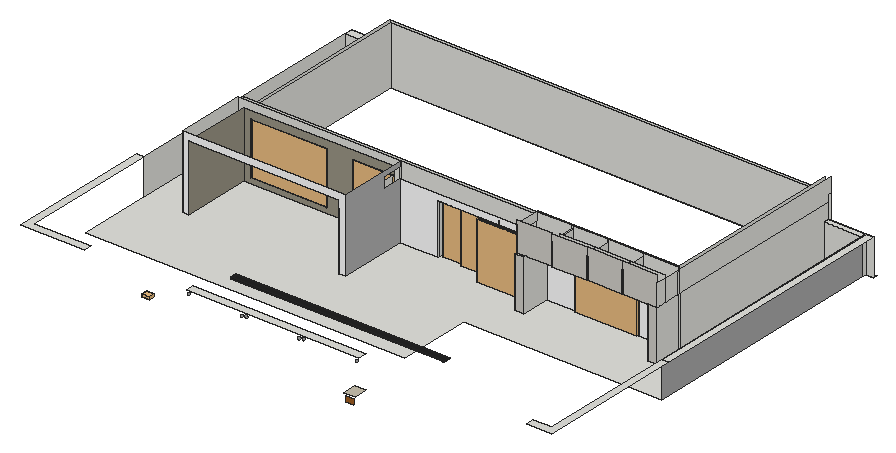
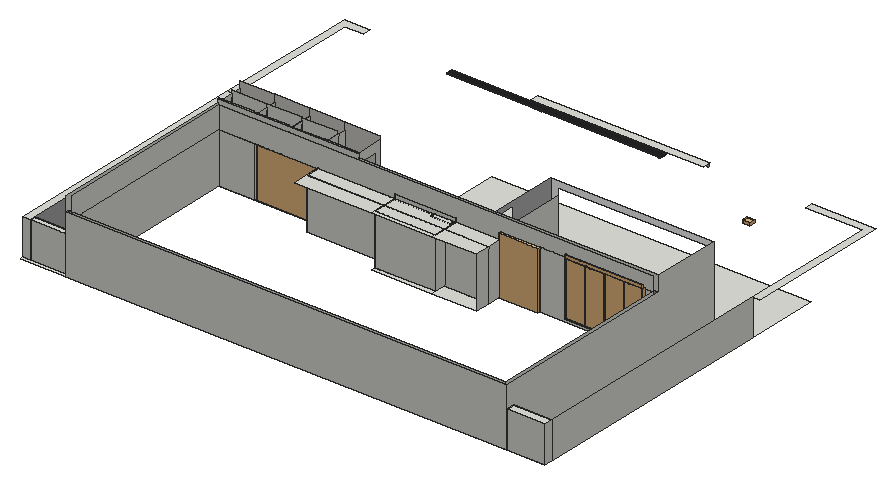
# SketchUp Ruby script. Lengths in inches.
U = 1.inch
M = Sketchup.active_model
def pt(a) = Geom::Point3d.new(a.map { |v| v * U })
def face(e, loops, mat)
  f = e.add_face(loops[0].map { |a| pt(a) })
  loops[1..].each { |l| e.add_face(l.map { |a| pt(a) }).erase! }
  f.material = f.back_material = mat if mat
  f
end
# faces: each face lists its corners as indices into pts; further lists are holes
def faces(e, pts, list, mat = nil) = list.each { |f| face(e, (f[0].is_a?(Array) ? f : [f]).map { |l| l.map { |i| pts[i] } }, mat) }
# xy, xz, yz: faces in a plane at the given z, y or x. An outline is a flat list of corners, or four numbers for a rectangle; further outlines are holes
def ring(l) = l.size == 4 ? [[l[0], l[1]], [l[2], l[1]], [l[2], l[3]], [l[0], l[3]]] : l.each_slice(2).to_a
def flat(e, list, mat, &to3) = list.each { |f| face(e, (f[0].is_a?(Array) ? f : [f]).map { |l| ring(l).map { |u, v| to3.(u, v) } }, mat) }
def xy(e, z, list, mat = nil) = flat(e, list, mat) { |x, y| [x, y, z] }
def xz(e, y, list, mat = nil) = flat(e, list, mat) { |x, z| [x, y, z] }
def yz(e, x, list, mat = nil) = flat(e, list, mat) { |y, z| [x, y, z] }
def lines(e, pts, list) = list.each { |a, b| e.add_line(pt(pts[a]), pt(pts[b])) }
# prism: a flat outline (further loops are holes) pulled along v
def prism(e, loops, v, mat = nil)
  f = face(e, loops, mat); d = Geom::Vector3d.new(v.map { |x| x * U })
  f.pushpull(f.normal.samedirection?(d) ? d.length : -d.length)
end
def box(e, o, s, mat = nil) = prism(e, [[o, [o[0] + s[0], o[1], o[2]], [o[0] + s[0], o[1] + s[1], o[2]], [o[0], o[1] + s[1], o[2]]]], [0, 0, s[2]], mat)
def at(x, y, z, deg = 0) = Geom::Transformation.translation(pt([x, y, z])) * Geom::Transformation.rotation(ORIGIN, Z_AXIS, deg.degrees)
def axes(o, x, y, z) = Geom::Transformation.new([*x, 0, *y, 0, *z, 0, *pt(o).to_a, 1])
def part(name) = M.definitions.add(name)
# library, detail: a bought-in or finely detailed component or shape, given as its bounding box
def library(name, o, s) = part(name).tap { |d| box(d.entities, o, s) }
def detail(e, o, s) = box(e.add_group.entities, o, s)
def put(e, d, t, mat = nil) = e.add_instance(d, t).tap { |i| i.material = mat if mat }
def group(e, t, mat = nil) = e.add_group.tap { |g| g.transformation = t; g.material = mat if mat }.entities
root = M.entities
M.materials.add("Material~3").color = [123, 113, 102]
M.materials.add("[0128_White]").color = [255, 255, 255]
M.materials.add("[0129_WhiteSmoke]").color = [178, 178, 178]
M.materials.add("[0132_LightGray]").color = [169, 169, 169]
M.materials.add("[0136_Charcoal]").color = [35, 35, 35]
M.materials.add("[Concrete Tile]").color = [155, 150, 134]
M.materials.add("[Terrazzo Tile Light]").color = [209, 207, 200]
M.materials.add("[Tile Canvas]").color = [199, 192, 173]
M.materials.add("[Wood Square Tile 02]").color = [160, 95, 34]
M.materials.add("terracota").color = [125, 74, 68]
c1 = library("3DGeom~4_Defintion",[362.52,-15.59,12.6],[288.85,70.11,1000])
c2 = library("3 door",[0,0,0],[74.8,3.9375,43.31])
c3 = library("Shallow planter bowl",[0,0,0],[21.33,16.65,7.48])
c4 = library("door (1)",[38.93,25.48,0],[40,9.94,82.68])
c5 = part("Group\#105")
prism(c5.entities,[[[353.71,0,0.79],[353.71,0,-1.18],[353.71,10.43,-1.18],[353.71,10.43,0.79],[353.71,10.12,0.79],[353.71,10.12,0.39],[353.71,7.09,0.39],[353.71,7.09,0.79],[353.71,6.73,0.79],[353.71,6.73,0.39],[353.71,3.7,0.39],[353.71,3.7,0.79],[353.71,3.35,0.79],[353.71,3.35,0.39],[353.71,0.31,0.39],[353.71,0.31,0.79]]],[-353.71,0,0])
c6 = library("JALI+PATTERN-03",[8.875,53.125,6.4375],[84,1,53.5])
xy(root,5.1875,[[[1168.49,611.53,1696.41,611.53,1696.41,732.28,2024.12,732.28,2024.12,1146.63,1960.87,1146.63,1960.87,851.0625,1791.45,851.0625,1791.45,845.35,1744,845.35,1744,798.41,1728.67,798.41,1728.67,845.35,1664.38,845.35,1664.38,874.25,1564.1,874.25,1564.1,845.35,1501.42,845.35,1501.42,732.28,1490.48,732.28,1490.48,851.0625,1425.1,851.0625,1425.1,845.35,1243.06,845.35,1243.06,732.28,1232.12,732.28,1232.12,1146.63,1168.49,1146.63],[1945.54,801.78,1960.87,845.35]],[1232.12,732.28,1232.12,1160.85,2036.12,1160.85,2036.12,1155.13,1237.84,1155.13,1237.84,851.0625,1425.1,851.0625,1425.1,845.35,1243.06,845.35,1243.06,732.28],[1490.48,732.28,1490.48,846.1,1564.1,846.1,1564.1,845.35,1501.42,845.35,1501.42,732.28],[1728.67,798.41,1728.67,845.35,1664.38,845.35,1664.38,846.1,1791.45,846.1,1791.45,845.35,1744,845.35,1744,798.41],[1945.54,801.78,1960.87,845.35],
  [1490.48,846.1,1564.1,874.25],[1664.38,846.1,1791.45,874.25],[1955.15,851.0625,1960.87,1155.13],[1490.48,874.25,1564.1,900.375],[1564.1,874.25,1664.38,892.35],
  [1564.1,892.35,1664.38,900.375],[1168.49,1146.63,1232.12,1160.85],[1960.87,1146.63,2024.12,1155.13]])
xy(root,13.84,[[1254.78,845.35,1379.65,851.0625]])
xy(root,32.74,[[1722.63,453.42,1741.07,475.99]],"[Tile Canvas]")
xy(root,65.1875,[[1156.87,491.47,1262.76,491.47,1262.76,505.1,1168.49,505.1,1168.49,732.28,1156.87,732.28],[1431.76,491.47,1716.62,505.1],[1993.42,491.47,2036.12,491.47,2036.12,732.28,2024.12,732.28,2024.12,505.1,1993.42,505.1],[2024.12,732.28,2036.12,1155.13],[1168.49,1146.63,1232.12,1160.85],
  [1960.87,1146.63,2024.12,1155.13]])
xy(root,89.42,[[1728.67,798.41,1744,801.78],[1744,801.78,1786.72,814.22],[1787.65,801.78,1791.45,817.6],[1791.45,801.78,1844.77,817.6],[1845.83,801.78,1896.07,817.6],
  [1896.07,801.78,1902.82,817.6],[1904.13,801.78,1945.54,817.6],[1945.54,801.78,1960.87,817.6],[1744,814.22,1786.72,844.47],[1787.65,817.6,1791.45,844.47],
  [1791.45,817.6,1844.77,844.47],[1845.83,817.6,1896.07,844.47],[1896.07,817.6,1902.82,844.47],[1904.13,817.6,1945.54,844.47],[1945.54,817.6,1960.87,844.47],
  [1728.67,844.47,1744,845.35],[1744,844.47,1791.45,845.35],[1791.45,844.47,1896.07,845.35],[1896.07,844.47,1945.54,845.35],[1945.54,844.47,1960.87,845.35],
  [1564.1,845.35,1664.38,846.1],[1664.38,845.35,1728.67,846.1],[1728.67,845.35,1791.45,846.1],[1791.45,845.35,1896.07,846.1],[1896.07,845.35,1960.87,846.1],
  [1490.48,846.1,1564.1,851.0625],[1664.38,846.1,1791.45,851.0625],[1791.45,846.1,1896.07,851.0625],[1896.07,846.1,1960.87,851.0625],[1490.48,851.0625,1564.1,874.25],
  [1564.1,851.0625,1664.38,874.25],[1664.38,851.0625,1791.45,874.25],[1955.15,851.0625,1960.87,1155.13],[1490.48,874.25,1564.1,900.375],[1564.1,874.25,1664.38,892.35],
  [1664.38,874.25,1791.45,900.375],[1564.1,892.35,1664.38,900.375]])
xz(root,453.42,[[1724.98,19.53,1739.11,29.34]],"[Wood Square Tile 02]")
xz(root,491.47,[[1522.98,57.74,1523.46,57.8,1523.92,57.99,1524.3,58.29,1524.6,58.68,1524.79,59.13,1524.85,59.61,1524.79,60.1,1524.6,60.55,1524.3,60.94,1523.92,61.24,1523.46,61.43,1522.98,61.49,1522.49,61.43,1522.04,61.24,1521.65,60.94,1521.36,60.55,1521.17,60.1,1521.1,59.61,1521.17,59.13,1521.36,58.68,1521.65,58.29,1522.04,57.99,1522.49,57.8],[1617.93,57.74,1618.41,57.8,1618.87,57.99,1619.26,58.29,1619.55,58.68,1619.74,59.13,1619.8,59.61,1619.74,60.1,1619.55,60.55,1619.26,60.94,1618.87,61.24,1618.41,61.43,1617.93,61.49,1617.44,61.43,1616.99,61.24,1616.6,60.94,1616.31,60.55,1616.12,60.1,1616.05,59.61,1616.12,59.13,1616.31,58.68,1616.6,58.29,1616.99,57.99,1617.44,57.8],[1712.88,57.74,1713.37,57.8,1713.82,57.99,1714.21,58.29,1714.5,58.68,1714.69,59.13,1714.76,59.61,1714.69,60.1,1714.5,60.55,1714.21,60.94,1713.82,61.24,1713.37,61.43,1712.88,61.49,1712.4,61.43,1711.94,61.24,1711.55,60.94,1711.26,60.55,1711.07,60.1,1711.01,59.61,1711.07,59.13,1711.26,58.68,1711.55,58.29,1711.94,57.99,1712.4,57.8],[1435.25,59.21,1435.73,59.22,1436.2,59.36,1436.62,59.61,1436.96,59.97,1437.19,60.4,1437.31,60.875,1437.3,61.36,1437.16,61.83,1436.9,62.25,1436.55,62.59,1436.12,62.82,1435.65,62.9375,1435.16,62.93,1434.6875,62.79,1434.27,62.53,1433.93,62.18,1433.7,61.75,1433.58,61.27,1433.59,60.78,1433.73,60.32,1433.99,59.9,1434.34,59.56,1434.77,59.33],[1530.2,59.21,1530.6875,59.22,1531.16,59.36,1531.57,59.61,1531.91,59.97,1532.15,60.4,1532.26,60.875,1532.25,61.36,1532.11,61.83,1531.86,62.25,1531.5,62.59,1531.07,62.82,1530.6,62.9375,1530.11,62.93,1529.64,62.79,1529.22,62.53,1528.88,62.18,1528.65,61.75,1528.53,61.27,1528.54,60.78,1528.68,60.32,1528.9375,59.9,1529.29,59.56,1529.72,59.33],
  [1625.15,59.21,1625.64,59.22,1626.11,59.36,1626.52,59.61,1626.86,59.97,1627.1,60.4,1627.21,60.875,1627.2,61.36,1627.0625,61.83,1626.81,62.25,1626.45,62.59,1626.02,62.82,1625.55,62.9375,1625.06,62.93,1624.59,62.79,1624.17,62.53,1623.83,62.18,1623.6,61.75,1623.48,61.27,1623.49,60.78,1623.63,60.32,1623.89,59.9,1624.24,59.56,1624.67,59.33]],"[0132_LightGray]")
xz(root,732.28,[[1232.12,5.1875,1243.06,5.1875,1243.06,114.25,1490.48,114.25,1490.48,5.1875,1501.42,5.1875,1501.42,125.1875,1232.12,125.1875]],"[0128_White]")
xz(root,798.41,[[1728.67,5.1875,1744,89.42]],"[Terrazzo Tile Light]")
xz(root,801.78,[[1945.54,5.1875,1960.87,89.42],[[1728.67,89.42,1786.72,138.0625],[1732.55,131.88,1732.26,131.92,1731.99,132.03,1731.76,132.21,1731.58,132.44,1731.47,132.71,1731.43,133,1731.47,133.29,1731.58,133.57,1731.76,133.8,1731.99,133.98,1732.26,134.09,1732.55,134.13,1732.84,134.09,1733.11,133.98,1733.35,133.8,1733.53,133.57,1733.64,133.29,1733.68,133,1733.64,132.71,1733.53,132.44,1733.35,132.21,1733.11,132.03,1732.84,131.92],[1783.68,131.88,1783.39,131.92,1783.11,132.03,1782.88,132.21,1782.7,132.44,1782.59,132.71,1782.55,133,1782.59,133.29,1782.7,133.57,1782.88,133.8,1783.11,133.98,1783.39,134.09,1783.68,134.13,1783.97,134.09,1784.24,133.98,1784.47,133.8,1784.65,133.57,1784.76,133.29,1784.8,133,1784.76,132.71,1784.65,132.44,1784.47,132.21,1784.24,132.03,1783.97,131.92],[1783.68,91.63,1783.39,91.67,1783.11,91.78,1782.88,91.96,1782.7,92.19,1782.59,92.46,1782.55,92.75,1782.59,93.04,1782.7,93.32,1782.88,93.55,1783.11,93.73,1783.39,93.84,1783.68,93.88,1783.97,93.84,1784.24,93.73,1784.47,93.55,1784.65,93.32,1784.76,93.04,1784.8,92.75,1784.76,92.46,1784.65,92.19,1784.47,91.96,1784.24,91.78,1783.97,91.67],[1731.49,91.63,1731.2,91.67,1730.93,91.78,1730.69,91.96,1730.52,92.19,1730.4,92.46,1730.36,92.75,1730.4,93.04,1730.52,93.32,1730.69,93.55,1730.93,93.73,1731.2,93.84,1731.49,93.88,1731.78,93.84,1732.05,93.73,1732.29,93.55,1732.46,93.32,1732.58,93.04,1732.61,92.75,1732.58,92.46,1732.46,92.19,1732.29,91.96,1732.05,91.78,1731.78,91.67]],[[1787.65,89.42,1844.77,138.0625],[1791.54,131.88,1791.25,131.92,1790.98,132.03,1790.74,132.21,1790.57,132.44,1790.45,132.71,1790.42,133,1790.45,133.29,1790.57,133.57,1790.74,133.8,1790.98,133.98,1791.25,134.09,1791.54,134.13,1791.83,134.09,1792.1,133.98,1792.34,133.8,1792.51,133.57,1792.63,133.29,1792.67,133,1792.63,132.71,1792.51,132.44,1792.34,132.21,1792.1,132.03,1791.83,131.92],[1842.67,91.63,1842.375,91.67,1842.1,91.78,1841.87,91.96,1841.69,92.19,1841.58,92.46,1841.54,92.75,1841.58,93.04,1841.69,93.32,1841.87,93.55,1842.1,93.73,1842.375,93.84,1842.67,93.88,1842.96,93.84,1843.23,93.73,1843.46,93.55,1843.64,93.32,1843.75,93.04,1843.79,92.75,1843.75,92.46,1843.64,92.19,1843.46,91.96,1843.23,91.78,1842.96,91.67],[1790.48,91.63,1790.1875,91.67,1789.92,91.78,1789.68,91.96,1789.5,92.19,1789.39,92.46,1789.35,92.75,1789.39,93.04,1789.5,93.32,1789.68,93.55,1789.92,93.73,1790.1875,93.84,1790.48,93.88,1790.77,93.84,1791.04,93.73,1791.27,93.55,1791.45,93.32,1791.56,93.04,1791.6,92.75,1791.56,92.46,1791.45,92.19,1791.27,91.96,1791.04,91.78,1790.77,91.67],[1842.67,131.88,1842.375,131.92,1842.1,132.03,1841.87,132.21,1841.69,132.44,1841.58,132.71,1841.54,133,1841.58,133.29,1841.69,133.57,1841.87,133.8,1842.1,133.98,1842.375,134.09,1842.67,134.13,1842.96,134.09,1843.23,133.98,1843.46,133.8,1843.64,133.57,1843.75,133.29,1843.79,133,1843.75,132.71,1843.64,132.44,1843.46,132.21,1843.23,132.03,1842.96,131.92]],[[1845.83,89.42,1902.82,138.0625],[1900.84,131.88,1900.55,131.92,1900.28,132.03,1900.05,132.21,1899.87,132.44,1899.75,132.71,1899.72,133,1899.75,133.29,1899.87,133.57,1900.05,133.8,1900.28,133.98,1900.55,134.09,1900.84,134.13,1901.13,134.09,1901.4,133.98,1901.64,133.8,1901.82,133.57,1901.93,133.29,1901.97,133,1901.93,132.71,1901.82,132.44,1901.64,132.21,1901.4,132.03,1901.13,131.92],[1849.72,131.88,1849.42,131.92,1849.15,132.03,1848.92,132.21,1848.74,132.44,1848.63,132.71,1848.59,133,1848.63,133.29,1848.74,133.57,1848.92,133.8,1849.15,133.98,1849.42,134.09,1849.72,134.13,1850.01,134.09,1850.28,133.98,1850.51,133.8,1850.69,133.57,1850.8,133.29,1850.84,133,1850.8,132.71,1850.69,132.44,1850.51,132.21,1850.28,132.03,1850.01,131.92],[1900.84,91.63,1900.55,91.67,1900.28,91.78,1900.05,91.96,1899.87,92.19,1899.75,92.46,1899.72,92.75,1899.75,93.04,1899.87,93.32,1900.05,93.55,1900.28,93.73,1900.55,93.84,1900.84,93.88,1901.13,93.84,1901.4,93.73,1901.64,93.55,1901.82,93.32,1901.93,93.04,1901.97,92.75,1901.93,92.46,1901.82,92.19,1901.64,91.96,1901.4,91.78,1901.13,91.67],[1848.65,91.63,1848.36,91.67,1848.09,91.78,1847.86,91.96,1847.68,92.19,1847.57,92.46,1847.53,92.75,1847.57,93.04,1847.68,93.32,1847.86,93.55,1848.09,93.73,1848.36,93.84,1848.65,93.88,1848.94,93.84,1849.22,93.73,1849.45,93.55,1849.63,93.32,1849.74,93.04,1849.78,92.75,1849.74,92.46,1849.63,92.19,1849.45,91.96,1849.22,91.78,1848.94,91.67]],[[1904.13,89.42,1960.87,138.0625],[1906.95,91.63,1906.66,91.67,1906.39,91.78,1906.16,91.96,1905.98,92.19,1905.87,92.46,1905.83,92.75,1905.87,93.04,1905.98,93.32,1906.16,93.55,1906.39,93.73,1906.66,93.84,1906.95,93.88,1907.25,93.84,1907.52,93.73,1907.75,93.55,1907.93,93.32,1908.04,93.04,1908.08,92.75,1908.04,92.46,1907.93,92.19,1907.75,91.96,1907.52,91.78,1907.25,91.67],[1908.02,131.88,1907.73,131.92,1907.45,132.03,1907.22,132.21,1907.04,132.44,1906.93,132.71,1906.89,133,1906.93,133.29,1907.04,133.57,1907.22,133.8,1907.45,133.98,1907.73,134.09,1908.02,134.13,1908.31,134.09,1908.58,133.98,1908.8125,133.8,1908.99,133.57,1909.1,133.29,1909.14,133,1909.1,132.71,1908.99,132.44,1908.8125,132.21,1908.58,132.03,1908.31,131.92],[1959.14,91.63,1958.85,91.67,1958.58,91.78,1958.35,91.96,1958.17,92.19,1958.06,92.46,1958.02,92.75,1958.06,93.04,1958.17,93.32,1958.35,93.55,1958.58,93.73,1958.85,93.84,1959.14,93.88,1959.43,93.84,1959.7,93.73,1959.9375,93.55,1960.12,93.32,1960.23,93.04,1960.27,92.75,1960.23,92.46,1960.12,92.19,1959.9375,91.96,1959.7,91.78,1959.43,91.67],[1959.14,131.88,1958.85,131.92,1958.58,132.03,1958.35,132.21,1958.17,132.44,1958.06,132.71,1958.02,133,1958.06,133.29,1958.17,133.57,1958.35,133.8,1958.58,133.98,1958.85,134.09,1959.14,134.13,1959.43,134.09,1959.7,133.98,1959.9375,133.8,1960.12,133.57,1960.23,133.29,1960.27,133,1960.23,132.71,1960.12,132.44,1959.9375,132.21,1959.7,132.03,1959.43,131.92]]],"[Terrazzo Tile Light]")
xz(root,817.6,[[1787.65,89.42,1844.77,131.1875],[1845.83,89.42,1902.82,131.1875],[1904.13,89.42,1960.87,131.1875]])
xz(root,844.47,[[1728.67,89.42,1786.72,131.1875],[1786.72,89.42,1787.65,131.1875],[1787.65,89.42,1844.77,131.1875],[1844.77,89.42,1845.83,131.1875],[1845.83,89.42,1902.82,131.1875],
  [1902.82,89.42,1904.13,131.1875],[1904.13,89.42,1960.87,131.1875]])
xz(root,845.35,[[1664.38,5.1875,1728.67,89.42],[1945.54,5.1875,1960.87,89.42]])
xz(root,845.35,[[1501.42,5.1875,1564.1,5.1875,1564.1,89.42,1728.67,89.42,1728.67,99.26,1501.42,99.26],[1744,5.1875,1791.45,89.42],[1896.07,5.1875,1945.54,89.42]],"[0128_White]")
xz(root,845.35,[[[1243.06,5.1875,1425.1,5.1875,1425.1,101.375,1490.48,101.375,1490.48,114.25,1243.06,114.25],[1254.78,13.84,1379.65,101.78]]],"[Concrete Tile]")
xz(root,846.1,[[1490.48,5.1875,1564.1,89.42],[1664.38,5.1875,1791.45,89.42],[1490.48,89.42,1501.42,89.42,1501.42,125.1875,1232.12,125.1875,1232.12,101.375,1490.48,101.375],[1501.42,89.42,1501.42,125.1875,1728.67,125.1875,1728.67,89.42,1664.38,89.42,1664.38,95.79,1564.1,95.79,1564.1,89.42],[1564.1,89.42,1664.38,95.79],
  [1728.67,89.42,1960.87,131.1875]])
xz(root,851.0625,[[1237.84,5.1875,1237.84,101.375,1254.78,101.375,1254.78,13.84,1379.65,13.84,1379.65,101.375,1425.1,101.375,1425.1,5.1875],[1896.07,5.1875,1955.15,89.42],[1955.15,5.1875,1960.87,89.42],[1490.48,89.42,1490.48,101.375,1379.65,101.375,1379.65,101.78,1254.78,101.78,1254.78,101.375,1237.84,101.375,1237.84,125.1875,1955.15,125.1875,1955.15,89.42,1664.38,89.42,1664.38,95.79,1564.1,95.79,1564.1,89.42],[1564.1,89.42,1664.38,95.79]])
xz(root,874.25,[[1490.48,5.1875,1791.45,89.42]])
xz(root,892.35,[[1564.1,5.1875,1664.38,89.42]])
xz(root,1146.63,[[1168.49,5.1875,1232.12,65.1875],[1960.87,5.1875,2024.12,65.1875]])
xz(root,1155.13,[[1237.84,5.1875,1955.15,101.375],[1955.15,5.1875,1960.87,89.42],[1960.87,5.1875,2024.12,65.1875],[2024.12,5.1875,2036.12,65.1875],[1955.15,89.42,1960.87,101.375]])
xz(root,1160.85,[[1168.49,5.1875,1232.12,65.1875],[1232.12,5.1875,1960.87,101.375]])
yz(root,1168.49,[[732.28,5.1875,1146.63,65.1875],[1146.63,5.1875,1160.85,65.1875]])
yz(root,1232.12,[[732.28,5.1875,732.28,125.1875,846.1,125.1875,846.1,101.375,1160.85,101.375,1160.85,65.1875,1146.63,65.1875,1146.63,5.1875],[1146.63,5.1875,1160.85,65.1875]])
yz(root,1237.84,[[851.0625,5.1875,1155.13,101.375]])
yz(root,1243.06,[[732.28,5.1875,845.35,114.25]],"[Concrete Tile]")
yz(root,1254.78,[[845.35,13.84,851.0625,101.78]])
yz(root,1379.65,[[845.35,13.84,851.0625,101.78]])
yz(root,1425.1,[[845.35,5.1875,851.0625,101.375]])
yz(root,1490.48,[[732.28,5.1875,846.1,101.375],[846.1,5.1875,874.25,89.42],[874.25,5.1875,900.375,89.42],[846.1,89.42,851.0625,101.375]])
yz(root,1501.42,[[845.35,89.42,846.1,125.1875]])
yz(root,1501.42,[[732.28,5.1875,845.35,5.1875,845.35,99.26,810.97,99.26,810.97,117.26,845.35,117.26,845.35,125.1875,732.28,125.1875]],"[0129_WhiteSmoke]")
yz(root,1564.1,[[845.35,5.1875,846.1,89.42],[846.1,5.1875,892.35,89.42],[846.1,89.42,851.0625,95.79]])
yz(root,1664.38,[[845.35,5.1875,846.1,89.42],[846.1,5.1875,892.35,89.42],[846.1,89.42,851.0625,95.79]])
yz(root,1728.67,[[798.41,5.1875,798.41,89.42,801.78,89.42,801.78,131.1875,844.47,131.1875,844.47,117.26,810.97,117.26,810.97,99.26,844.47,99.26,844.47,89.42,845.35,89.42,845.35,5.1875],[844.47,89.42,845.35,99.26],[845.35,89.42,846.1,125.1875]])
yz(root,1744,[[798.41,5.1875,845.35,89.42]])
yz(root,1786.72,[[801.78,89.42,814.22,125.1875],[814.22,89.42,844.47,125.1875]])
yz(root,1787.65,[[801.78,89.42,817.6,125.1875],[817.6,89.42,844.47,125.1875]])
yz(root,1791.45,[[845.35,5.1875,846.1,89.42],[846.1,5.1875,874.25,89.42]])
yz(root,1844.77,[[801.78,89.42,817.6,125.1875],[817.6,89.42,844.47,125.1875]])
yz(root,1845.83,[[801.78,89.42,817.6,125.1875],[817.6,89.42,844.47,125.1875]])
yz(root,1896.07,[[845.35,5.1875,851.0625,89.42]])
yz(root,1902.82,[[801.78,89.42,817.6,125.1875],[817.6,89.42,844.47,125.1875]])
yz(root,1904.13,[[801.78,89.42,817.6,125.1875],[817.6,89.42,844.47,125.1875]])
yz(root,1945.54,[[801.78,5.1875,845.35,89.42]])
yz(root,1955.15,[[851.0625,5.1875,1155.13,89.42],[851.0625,89.42,1155.13,125.1875]])
yz(root,1960.87,[[801.78,5.1875,845.35,89.42],[851.0625,5.1875,1146.63,5.1875,1146.63,65.1875,1155.13,65.1875,1155.13,89.42,851.0625,89.42],[1146.63,5.1875,1155.13,65.1875],[801.78,89.42,817.6,125.1875],[817.6,89.42,844.47,125.1875],
  [844.47,89.42,846.1,125.1875],[846.1,89.42,1155.13,89.42,1155.13,101.375,1160.85,101.375,1160.85,125.1875,846.1,125.1875]])
yz(root,2024.12,[[1146.63,5.1875,1155.13,65.1875]])
yz(root,2024.12,[[732.28,5.1875,1146.63,65.1875]],"[0132_LightGray]")
p = [[1728.67,814.22,89.42],[1744,814.22,89.42]]
lines(root,p,[[0,1]])
put(root,c1,axes([1212.17,853.3125,12.94],[0.11056,0,0],[0,-0.05859,0],[0,0,0.08734]),"Material~3")
put(root,c1,axes([1243.65,853.99,12.94],[0.11056,0,0],[0,-0.05859,0],[0,0,0.08734]),"Material~3")
put(root,c2,axes([1254.78,847.72,10.15],[1.71563,0,0],[0,1.38,0],[0,0,2.21476]))
put(root,c1,axes([1275.71,853.99,12.94],[0.11056,0,0],[0,-0.05859,0],[0,0,0.08734]),"Material~3")
put(root,c3,axes([1355.09,510.84,16.37],[-0.59053,0,0],[0,0.56886,0],[0,0,0.56886]),"terracota")
put(root,c1,axes([1307.77,853.99,12.94],[0.11056,0,0],[0,-0.05859,0],[0,0,0.08734]),"Material~3")
put(root,c4,axes([1361.48,814.19,5.1875],[1.63437,0,0],[0,1.16,0],[0,0,1.16]))
put(root,c1,axes([1527.06,857.09,3.96],[0.11056,0,0],[0,-0.11056,0],[0,0,0.08439]),"Material~3")
put(root,c1,axes([1560.43,851.7,3.96],[0.11056,0,0],[0,-0.08955,0],[0,0,0.08439]),"Material~3")
put(root,c1,axes([1592.37,851.7,3.96],[0.11056,0,0],[0,-0.08955,0],[0,0,0.08439]),"Material~3")
put(root,c5,axes([1473.09,541.01,81.03],[1,0,0],[0,-1,0],[0,0,-1]),"[0136_Charcoal]")
put(root,c6,axes([1634.01,766.91,109.2],[0,0,-1.12],[0,1.12,0],[1.5792,0,0]))
put(root,c2,axes([1791.45,843.85,5.1875],[1.38,0,0],[0,1.38,0],[0,0,1.94496]))
